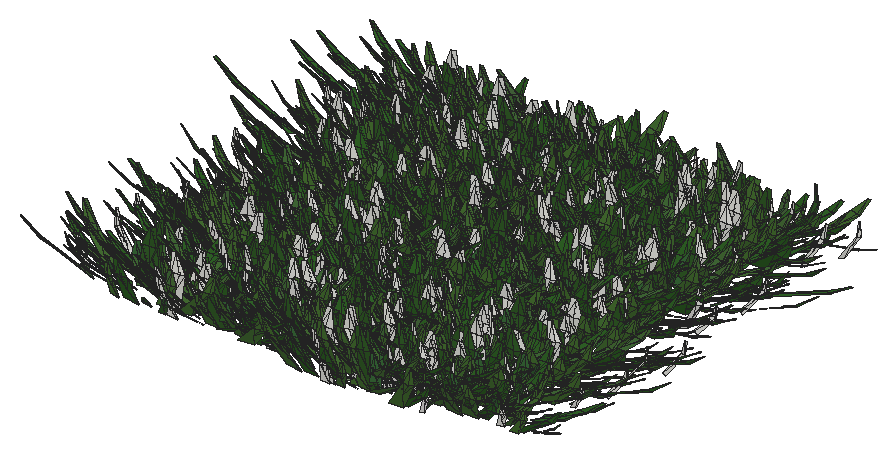
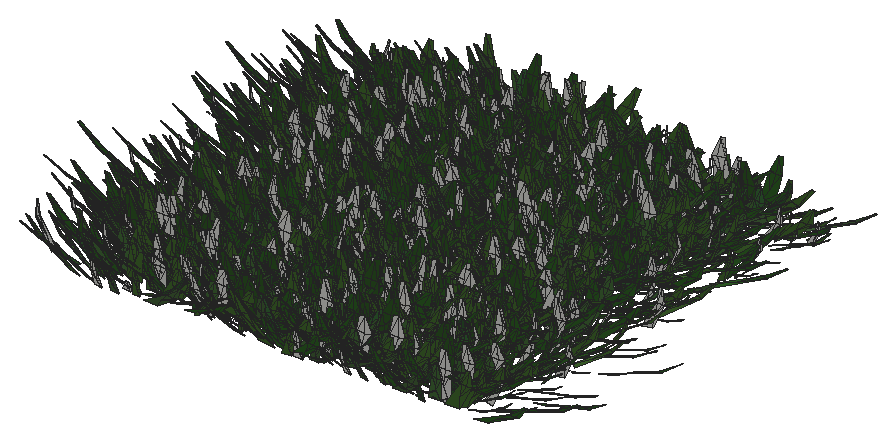
# SketchUp Ruby script. Lengths in inches.
U = 1.inch
M = Sketchup.active_model
def pt(a) = Geom::Point3d.new(a.map { |v| v * U })
def face(e, loops, mat)
  f = e.add_face(loops[0].map { |a| pt(a) })
  loops[1..].each { |l| e.add_face(l.map { |a| pt(a) }).erase! }
  f.material = f.back_material = mat if mat
  f
end
# faces: each face lists its corners as indices into pts; further lists are holes
def faces(e, pts, list, mat = nil) = list.each { |f| face(e, (f[0].is_a?(Array) ? f : [f]).map { |l| l.map { |i| pts[i] } }, mat) }
# xy, xz, yz: faces in a plane at the given z, y or x. An outline is a flat list of corners, or four numbers for a rectangle; further outlines are holes
def ring(l) = l.size == 4 ? [[l[0], l[1]], [l[2], l[1]], [l[2], l[3]], [l[0], l[3]]] : l.each_slice(2).to_a
def flat(e, list, mat, &to3) = list.each { |f| face(e, (f[0].is_a?(Array) ? f : [f]).map { |l| ring(l).map { |u, v| to3.(u, v) } }, mat) }
def xy(e, z, list, mat = nil) = flat(e, list, mat) { |x, y| [x, y, z] }
def xz(e, y, list, mat = nil) = flat(e, list, mat) { |x, z| [x, y, z] }
def yz(e, x, list, mat = nil) = flat(e, list, mat) { |y, z| [x, y, z] }
def lines(e, pts, list) = list.each { |a, b| e.add_line(pt(pts[a]), pt(pts[b])) }
# prism: a flat outline (further loops are holes) pulled along v
def prism(e, loops, v, mat = nil)
  f = face(e, loops, mat); d = Geom::Vector3d.new(v.map { |x| x * U })
  f.pushpull(f.normal.samedirection?(d) ? d.length : -d.length)
end
def box(e, o, s, mat = nil) = prism(e, [[o, [o[0] + s[0], o[1], o[2]], [o[0] + s[0], o[1] + s[1], o[2]], [o[0], o[1] + s[1], o[2]]]], [0, 0, s[2]], mat)
def at(x, y, z, deg = 0) = Geom::Transformation.translation(pt([x, y, z])) * Geom::Transformation.rotation(ORIGIN, Z_AXIS, deg.degrees)
def axes(o, x, y, z) = Geom::Transformation.new([*x, 0, *y, 0, *z, 0, *pt(o).to_a, 1])
def part(name) = M.definitions.add(name)
# library, detail: a bought-in or finely detailed component or shape, given as its bounding box
def library(name, o, s) = part(name).tap { |d| box(d.entities, o, s) }
def detail(e, o, s) = box(e.add_group.entities, o, s)
def put(e, d, t, mat = nil) = e.add_instance(d, t).tap { |i| i.material = mat if mat }
def group(e, t, mat = nil) = e.add_group.tap { |g| g.transformation = t; g.material = mat if mat }.entities
root = M.entities
M.materials.add("Material10").color = [48, 100, 38]
M.materials.add("Material3").color = [68, 110, 58]
M.materials.add("Material4").color = [48, 90, 38]
M.materials.add("Material5").color = [68, 110, 48]
M.materials.add("Material6").color = [48, 90, 48]
M.materials.add("Material7").color = [58, 110, 58]
M.materials.add("Material8").color = [58, 90, 38]
M.materials.add("Material9").color = [68, 100, 58]
c1 = part("grass00")
p = [[-0.6875,0.15,0],[-0.56,0.08,5.52],[-0.04,0.03,2.76],[0.48,-0.02,0],[0.35,-0.02,5.52],[-0.1,-0.14,5.52],
  [-0.12,0.65,8.37],[-0.42,0.65,8.37]]
faces(c1.entities,p,[[0,1,2,3],[3,2,4],[1,5,2],[5,4,2],[1,6,5],[4,5,6],[7,6,1]])
c2 = part("Group16\#1")
put(c2.entities,c1,axes([1.44,-0.61,-0.01],[0.05352,0.12609,0],[-0.10704,0.04543,0.07239],[0.06664,-0.02828,0.11628]),"Material6")
put(c2.entities,c1,axes([0.76,-0.15,-0.01],[0.04676,0.24062,0],[-0.23162,0.04501,0.06642],[0.0652,-0.01267,0.23595]),"Material3")
put(c2.entities,c1,axes([0.79,0.01,-0.01],[-0.00606,0.34651,0],[-0.34381,-0.00602,0.0432],[0.04319,0.00076,0.34386]))
put(c2.entities,c1,axes([1,0.23,-0.01],[-0.07192,0.31144,0],[-0.28722,-0.06632,0.1236],[0.12043,0.02781,0.29478]),"Material5")
put(c2.entities,c1,axes([1.66,0.77,-0.01],[-0.13828,0.29651,0],[-0.21551,-0.1005,0.22471],[0.20365,0.09498,0.23779]),"Material10")
put(c2.entities,c1,axes([0.6875,0.52,-0.01],[-0.18126,0.24051,0],[-0.22746,-0.17142,0.09788],[0.07817,0.05891,0.28481]),"Material5")
put(c2.entities,c1,axes([0.68,0.78,-0.01],[-0.215,0.18688,0],[-0.12385,-0.14248,0.21334],[0.13995,0.16101,0.18878]),"Material3")
put(c2.entities,c1,axes([0.56,1,-0.01],[-0.13756,0.07624,0],[-0.06159,-0.11112,0.0927],[0.04494,0.08108,0.12705]),"Material5")
put(c2.entities,c1,axes([0.2,0.64,-0.01],[-0.23729,0.07254,0],[-0.05711,-0.18681,0.153],[0.04473,0.14632,0.19535]),"Material10")
put(c2.entities,c1,axes([0.0625,0.72,-0.01],[-0.28874,0.02525,0],[-0.02179,-0.24916,0.14647],[0.01276,0.14591,0.25012]),"Material3")
put(c2.entities,c1,axes([-0.08,0.62,-0.01],[-0.34089,-0.04187,0],[0.03255,-0.26504,0.216],[-0.02633,0.21439,0.26703]),"Material10")
put(c2.entities,c1,axes([-0.34,0.98,-0.01],[-0.14314,-0.0493,0],[0.04397,-0.12769,0.06843],[-0.02228,0.0647,0.13505]),"Material10")
put(c2.entities,c1,axes([-0.87,1.45,-0.01],[-0.23488,-0.14114,0],[0.13761,-0.22901,0.06087],[-0.03135,0.05217,0.26717]))
put(c2.entities,c1,axes([-0.72,0.77,-0.01],[-0.14208,-0.13251,0],[0.07209,-0.0773,0.16301],[-0.11118,0.11922,0.1057]),"Material10")
put(c2.entities,c1,axes([-0.62,0.43,-0.01],[-0.14845,-0.21203,0],[0.18654,-0.13061,0.12304],[-0.10079,0.07057,0.22772]),"Material3")
put(c2.entities,c1,axes([-0.68,0.29,-0.01],[-0.13639,-0.32136,0],[0.31723,-0.13464,0.05579],[-0.05136,0.0218,0.34462]),"Material4")
put(c2.entities,c1,axes([-0.64,0.125,-0.01],[-0.0458,-0.23569,0],[0.22124,-0.043,0.08276],[-0.08124,0.01579,0.22538]),"Material7")
put(c2.entities,c1,axes([-1.6,-0.03,-0.01],[0.00576,-0.32897,0],[0.27526,0.00482,0.18018],[-0.18015,-0.00315,0.2753]),"Material5")
put(c2.entities,c1,axes([-1.36,-0.31,-0.01],[0.05718,-0.24765,0],[0.18172,0.04196,0.17267],[-0.16825,-0.03885,0.1865]),"Material10")
put(c2.entities,c1,axes([-1.54,-0.72,-0.01],[0.06537,-0.14017,0],[0.13555,0.06321,0.03939],[-0.0357,-0.01665,0.14956]))
put(c2.entities,c1,axes([-1.19,-0.9,-0.01],[0.09597,-0.12735,0],[0.11214,0.08451,0.07557],[-0.06035,-0.04548,0.14042]),"Material9")
put(c2.entities,c1,axes([-0.47,-0.54,-0.01],[0.11588,-0.10072,0],[0.0618,0.0711,0.12124],[-0.07953,-0.0915,0.0942]))
put(c2.entities,c1,axes([-0.47,-0.84,-0.01],[0.11927,-0.0661,0],[0.06603,0.11913,0.00646],[-0.00313,-0.00565,0.13621]),"Material5")
put(c2.entities,c1,axes([-0.38,-1.24,-0.01],[0.28037,-0.08571,0],[0.0618,0.20215,0.20315],[-0.05939,-0.19428,0.21139]),"Material9")
put(c2.entities,c1,axes([-0.06,-0.66,-0.01],[0.22719,-0.01987,0],[0.01247,0.14255,0.17758],[-0.01547,-0.17691,0.1431]),"Material8")
put(c2.entities,c1,axes([0.11,-0.89,-0.01],[0.14882,0.01828,0],[-0.01058,0.08611,0.12229],[0.01491,-0.12138,0.08676]),"Material6")
put(c2.entities,c1,axes([0.25,-0.72,-0.01],[0.20481,0.07053,0],[-0.06206,0.18022,0.10291],[0.03351,-0.0973,0.1906]),"Material6")
put(c2.entities,c1,axes([0.85,-1.42,-0.01],[0.16481,0.09904,0],[-0.09472,0.15762,0.05616],[0.02893,-0.04814,0.18389]),"Material5")
put(c2.entities,c1,axes([1.01,-1.09,-0.01],[0.21858,0.20385,0],[-0.17495,0.1876,0.15339],[0.10462,-0.11218,0.25652]),"Material10")
put(c2.entities,c1,axes([1.01,-0.71,-0.01],[0.08733,0.12473,0],[-0.06445,0.04512,0.13037],[0.1068,-0.07477,0.07867]),"Material6")
c3 = part("Group15\#1")
put(c3.entities,c2,at(0,0,0))
c4 = part("3darcstudiotree_grass00\#1")
put(c4.entities,c3,at(0,0,0))
put(root,c4,axes([26.17,52.48,7.6],[-3.35209,-0.40812,0],[1.8256,-0.93715,-0.03924],[0.12725,-0.06532,1.93013]))
put(root,c4,axes([26.28,43.875,7.6],[3.10625,-0.85798,0],[3.45102,0.78089,-0.01132],[0.05281,0.01195,1.83032]))
put(root,c4,axes([27.35,67.6875,7.6],[0.47327,-1.08686,0],[4.60722,0.12539,-0.01362],[0.07238,0.00197,1.54899]))
put(root,c4,axes([26.83,70.39,7.6],[-3.67097,0.66942,0],[-2.79157,-0.95678,-0.03459],[-0.12687,-0.04348,1.84283]))
put(root,c4,axes([27.96,75.08,7.6],[-1.67308,-0.99744,0],[3.57228,-0.3745,-0.00949],[0.05914,-0.0062,1.63563]))
put(root,c4,axes([26.8,76.65,7.6],[-2.74123,0.86634,0],[-3.57969,-0.70792,-0.0328],[-0.11955,-0.02364,1.32564]))
put(root,c4,axes([27.89,55.68,7.6],[-4.42043,-0.11266,0],[0.48566,-1.19101,-0.03002],[0.01626,-0.03988,1.59842]))
put(root,c4,axes([27.0625,81.24,7.6],[-1.61796,0.93996,0],[-3.84011,-0.41313,-0.01574],[-0.09207,-0.00991,1.66349]))
put(root,c4,axes([27.55,59.01,7.6],[3.17321,-0.79133,0],[2.66412,0.66769,-0.0036],[0.01703,0.00427,1.5794]))
put(root,c4,axes([26.68,71.74,7.6],[3.39555,0.33213,0],[-1.83469,1.1723,-0.03882],[-0.07009,0.04479,1.55956]))
put(root,c4,axes([27.8,79.22,7.6],[-2.84065,0.70186,0],[-3.36417,-0.85098,-0.01852],[-0.06548,-0.01656,1.50457]))
put(root,c4,axes([27.46,46.76,7.6],[4.32578,-0.20958,0],[0.90693,1.16992,-0.01483],[0.01432,0.01847,1.51152]))
put(root,c4,axes([27.13,61.86,7.6],[3.67456,0.57849,0],[-2.21589,0.8797,-0.03908],[-0.14607,0.05799,1.82303]))
put(root,c4,axes([27.9375,50.86,7.6],[3.12654,0.99148,0],[-3.05993,0.60307,-0.04305],[-0.21095,0.04158,1.51958]))
put(root,c4,axes([30.63,76.96,7.6],[-3.92204,-0.29054,0],[1.17803,-0.99389,-0.05017],[0.08482,-0.07156,1.54202]))
put(root,c4,axes([31.09,70.53,7.6],[-2.30872,-1.02741,0],[3.84342,-0.53979,-0.0488],[0.20495,-0.02878,1.32723]))
put(root,c4,axes([29.8,66.42,7.6],[4.53918,0.22078,0],[-0.91725,1.17863,-0.03864],[-0.04554,0.05852,1.85268]))
put(root,c4,axes([30.03,44.67,7.6],[4.62634,0.00391,0],[-0.01264,0.9349,-0.00416],[-0.00008,0.00596,1.3392]))
put(root,c4,axes([29.99,46.42,7.6],[3.44705,0.83738,0],[-3.43715,0.8843,-0.06236],[-0.26248,0.06753,1.86199]))
put(root,c4,axes([31.96,81.48,7.6],[-2.93,-0.68293,0],[3.05684,-0.81968,-0.04642],[0.17067,-0.04577,1.51042]))
put(root,c4,axes([31.44,64.16,7.6],[1.34292,-0.85261,0],[4.14174,0.40772,-0.0431],[0.19924,0.01961,1.38217]))
put(root,c4,axes([31.49,55.18,7.6],[2.29787,-0.71294,0],[3.86866,0.77932,-0.04335],[0.16802,0.03385,1.54559]))
put(root,c4,axes([32.17,75.38,7.6],[-1.22669,-1.03547,0],[3.63714,-0.2693,-0.01669],[0.12283,-0.00909,1.82011]))
put(root,c4,axes([31.35,52.72,7.6],[-2.98365,0.86497,0],[-3.89047,-0.83874,-0.04683],[-0.20597,-0.0444,1.86493]))
put(root,c4,axes([32.55,73.4,7.6],[-4.10256,-0.1973,0],[0.74416,-0.9671,-0.01319],[0.01782,-0.02316,1.76124]))
put(root,c4,axes([30.78,56.9,7.6],[4.13068,0.36881,0],[-1.71772,1.2024,-0.02984],[-0.04889,0.03422,1.55474]))
put(root,c4,axes([32.57,54.03,7.6],[0.7791,-0.92292,0],[4.72913,0.24951,-0.04294],[0.18667,0.00985,1.34209]))
put(root,c4,axes([33.16,77.8,7.6],[-4.4686,-0.23956,0],[0.88176,-1.02798,-0.03168],[0.03699,-0.04313,1.46389]))
put(root,c4,axes([32.88,58.94,7.6],[1.878,-0.85136,0],[4.01986,0.55421,-0.00061],[0.00361,0.0005,1.94394]))
put(root,c4,axes([33.25,60.34,7.6],[1.24313,-0.92825,0],[4.47227,0.37433,-0.04023],[0.17657,0.01478,1.36415]))
put(root,c4,axes([32.24,63.11,7.6],[-2.14811,0.98739,0],[-4.23231,-0.57547,-0.01158],[-0.04996,-0.00679,1.47884]))
put(root,c4,axes([33.77,67.41,7.6],[-0.51909,-1.27053,0],[4.17352,-0.10657,-0.01024],[0.07103,-0.00181,1.82793]))
put(root,c4,axes([33.17,43.86,7.6],[-2.15627,0.7748,0],[-3.75013,-0.65229,-0.02835],[-0.11927,-0.02075,1.46355]))
put(root,c4,axes([32.47,69.33,7.6],[-0.2443,0.90017,0],[-4.80232,-0.08146,-0.00038],[-0.00184,-0.00003,1.44006]))
put(root,c4,axes([32.82,71.58,7.6],[3.055,0.70222,0],[-2.89109,0.7861,-0.04265],[-0.20546,0.05586,1.90027]))
put(root,c4,axes([33.14,61.48,7.6],[-2.4391,1.11365,0],[-4.52145,-0.61893,-0.00813],[-0.02921,-0.004,1.31962]))
put(root,c4,axes([33.52,50.68,7.6],[-2.85701,0.97241,0],[-3.78392,-0.69484,-0.02364],[-0.12588,-0.02312,1.93862]))
put(root,c4,axes([33.93,49.92,7.6],[3.76686,-0.83119,0],[3.36509,0.95314,-0.00351],[0.01175,0.00333,1.60808]))
put(root,c4,axes([33.96,48.31,7.6],[2.81917,-0.76619,0],[3.32904,0.76557,-0.05921],[0.2958,0.06802,1.91907]))
put(root,c4,axes([33.97,79.74,7.6],[-2.30663,1.06552,0],[-4.23551,-0.57306,-0.04902],[-0.25303,-0.03424,1.76654]))
put(root,c4,axes([36.06,61.82,7.6],[-1.10466,-1.04309,0],[4.11781,-0.27255,-0.00114],[0.00731,-0.00048,1.77079]))
put(root,c4,axes([36.38,52.53,7.6],[-4.80824,-0.47237,0],[1.62347,-1.03284,-0.03326],[0.06769,-0.04306,1.54402]))
put(root,c4,axes([36.37,62.78,7.6],[-4.86512,0.05083,0],[-0.1686,-1.00853,-0.02048],[-0.00677,-0.04048,1.99696]))
put(root,c4,axes([35.83,59.86,7.6],[-3.02468,0.58391,0],[-2.63511,-0.85312,-0.02049],[-0.06609,-0.0214,1.42185]))
put(root,c4,axes([36.38,70.74,7.6],[2.33832,-0.89865,0],[3.29868,0.53645,-0.01966],[0.11007,0.0179,1.64285]))
put(root,c4,axes([37.07,76.47,7.6],[-3.01459,0.57554,0],[-2.90712,-0.95168,-0.0597],[-0.23401,-0.07661,1.93343]))
put(root,c4,axes([36.58,80.09,7.6],[-1.87724,0.90474,0],[-4.04075,-0.52401,-0.04385],[-0.19356,-0.0251,1.41492]))
put(root,c4,axes([37.13,71.88,7.6],[-2.76695,1.05816,0],[-3.42506,-0.55976,-0.05029],[-0.32743,-0.05351,1.98932]))
put(root,c4,axes([37.48,68.93,7.6],[1.10502,-1.02921,0],[4.51643,0.30307,-0.05256],[0.2763,0.01854,1.59089]))
put(root,c4,axes([37.96,75.13,7.6],[-0.89548,-0.9705,0],[4.23678,-0.24433,-0.03351],[0.19208,-0.01108,1.59864]))
put(root,c4,axes([36.48,47.99,7.6],[4.62222,-0.11265,0],[0.48715,1.24932,-0.00515],[0.00288,0.00739,1.80879]))
put(root,c4,axes([38.8,45.89,7.6],[-4.55832,-0.10477,0],[0.39974,-1.08695,-0.01686],[0.00782,-0.02126,1.38194]))
put(root,c4,axes([37.36,57.46,7.6],[-0.72748,0.92095,0],[-4.90606,-0.24221,-0.01512],[-0.08825,-0.00436,1.85999]))
put(root,c4,axes([39.07,51.3125,7.6],[1.03269,-0.98427,0],[4.16593,0.27318,-0.01105],[0.06051,0.00397,1.52421]))
put(root,c4,axes([37.49,44.97,7.6],[1.02056,1.16632,0],[-3.98079,0.21771,-0.00261],[-0.01671,0.00091,1.6704]))
put(root,c4,axes([37.49,67.8,7.6],[2.79724,0.70196,0],[-3.39919,0.84659,-0.03194],[-0.10291,0.02563,1.36388]))
put(root,c4,axes([39.77,55.68,7.6],[-4.31262,-0.5264,0],[2.25127,-1.15275,-0.06565],[0.15274,-0.07821,1.70067]))
put(root,c4,axes([39.99,81.44,7.6],[-1.35682,-1.23326,0],[4.57935,-0.31489,-0.02011],[0.12844,-0.00883,1.9663]))
put(root,c4,axes([38.01,58.25,7.6],[-0.08255,1.17083,0],[-4.86044,-0.02142,-0.00958],[-0.04676,-0.00021,1.48335]))
put(root,c4,axes([38.42,73.11,7.6],[4.4348,0.59016,0],[-2.24354,1.0537,-0.02998],[-0.09351,0.04392,1.98098]))
put(root,c4,axes([38.92,49.8125,7.6],[0.34603,1.04205,0],[-3.81852,0.07925,-0.00998],[-0.05603,0.00116,1.34846]))
put(root,c4,axes([39.82,66.52,7.6],[3.30812,-0.80284,0],[2.65209,0.683,-0.02978],[0.12492,0.03217,1.43312]))
put(root,c4,axes([39.22,64.0625,7.6],[3.9282,0.38594,0],[-1.52945,0.97295,-0.02634],[-0.05842,0.03716,1.58474]))
put(root,c4,axes([39.91,53.36,7.6],[3.43387,-0.66059,0],[2.3393,0.76,-0.03629],[0.13053,0.04241,1.41389]))
put(root,c4,axes([40.05,78.42,7.6],[3.76187,0.14522,0],[-0.63051,1.02078,-0.03647],[-0.03383,0.05478,1.56991]))
put(root,c4,axes([41.96,65.59,7.6],[-4.18758,-0.22232,0],[0.96219,-1.13271,-0.02543],[0.02933,-0.03453,1.60712]))
put(root,c4,axes([42.84,61.76,7.6],[-1.50965,-1.02726,0],[3.51869,-0.32319,-0.02344],[0.12593,-0.01157,1.34096]))
put(root,c4,axes([42.66,82.25,7.6],[-4.14711,0.13047,0],[-0.48074,-0.95501,-0.01354],[-0.00996,-0.01978,1.41676]))
put(root,c4,axes([42.59,49.45,7.6],[-3.93065,0.22936,0],[-0.83099,-0.89006,-0.0198],[-0.02909,-0.03116,1.47686]))
put(root,c4,axes([42.41,62.96,7.6],[1.12797,-1.08226,0],[3.79109,0.24695,-0.04641],[0.27021,0.0176,1.47323]))
put(root,c4,axes([43.23,59.81,7.6],[0.07706,-1.18991,0],[5.14858,0.02084,-0.02796],[0.13847,0.00056,1.59394]))
put(root,c4,axes([43.34,58.04,7.6],[-4.65628,0.436,0],[-1.28176,-0.85553,-0.01358],[-0.03081,-0.02057,1.47772]))
put(root,c4,axes([43.74,56.96,7.6],[-4.55351,-0.01078,0],[0.04878,-1.28737,-0.04475],[0.00189,-0.04985,1.43393]))
put(root,c4,axes([43.03,67.88,7.6],[3.27668,-0.61327,0],[2.78187,0.92896,-0.01707],[0.06911,0.02308,1.96039]))
put(root,c4,axes([43.96,55.76,7.6],[-4.03083,-0.21133,0],[0.96222,-1.14709,-0.00999],[0.00968,-0.01153,1.38276]))
put(root,c4,axes([42.52,73.625,7.6],[4.2465,-0.26624,0],[0.87998,0.87721,-0.03452],[0.06922,0.06901,1.86367]))
put(root,c4,axes([43.5625,65.09,7.6],[-2.58663,0.93393,0],[-3.19563,-0.55317,-0.03104],[-0.18757,-0.03247,1.78553]))
put(root,c4,axes([44.08,47.88,7.6],[3.25384,-0.82472,0],[2.88656,0.71179,-0.00165],[0.00841,0.00207,1.81884]))
put(root,c4,axes([43.29,71.82,7.6],[4.50216,0.32859,0],[-1.15691,0.9907,-0.03197],[-0.04777,0.04091,1.37583]))
put(root,c4,axes([45.35,79.77,7.6],[-3.56236,-0.42367,0],[2.09245,-1.09962,-0.03826],[0.09877,-0.05191,1.82966]))
put(root,c4,axes([45.22,44.79,7.6],[-1.82775,-1.1638,0],[4.23116,-0.41531,-0.05278],[0.32118,-0.03153,1.85719]))
put(root,c4,axes([45.34,45.84,7.6],[-4.77315,-0.10069,0],[0.4015,-1.18962,-0.02802],[0.01422,-0.04212,1.8014]))
put(root,c4,axes([43.91,53.65,7.6],[4.00974,0.00197,0],[-0.00725,0.92038,-0.0306],[-0.0005,0.06325,1.9022]))
put(root,c4,axes([45.46,52.69,7.6],[-3.72919,-0.05138,0],[0.24763,-1.12327,-0.00601],[0.00211,-0.00957,1.79325]))
put(root,c4,axes([45.55,76.17,7.6],[1.19738,-1.09661,0],[4.52965,0.30912,-0.00598],[0.02664,0.00182,1.35627]))
put(root,c4,axes([44.76,75.65,7.6],[3.65568,-0.70914,0],[2.22099,0.71559,-0.00126],[0.00457,0.00147,1.3431]))
put(root,c4,axes([45.16,80.75,7.6],[2.61731,-0.86986,0],[3.89148,0.73181,-0.05537],[0.21942,0.04126,1.50911]))
put(root,c4,axes([44.58,77.9375,7.6],[3.93859,-0.14638,0],[0.69101,1.16209,-0.00967],[0.00686,0.01153,1.41667]))
put(root,c4,axes([44.36,43.44,7.6],[1.45046,1.05694,0],[-4.51111,0.38692,-0.02597],[-0.16209,0.0139,1.96681]))
put(root,c4,axes([44.36,51.22,7.6],[3.4597,0.79761,0],[-3.28778,0.89131,-0.03053],[-0.13377,0.03626,1.95907]))
put(root,c4,axes([45.58,70.75,7.6],[-2.65201,0.65355,0],[-3.42376,-0.86832,-0.05994],[-0.20928,-0.05308,1.51606]))
put(root,c4,axes([44.67,69.22,7.6],[2.03961,1.07438,0],[-3.7474,0.44463,-0.01135],[-0.07143,0.00848,1.80626]))
put(root,c4,axes([48.18,69.59,7.6],[-4.36276,-0.41418,0],[1.61781,-1.06507,-0.04397],[0.10568,-0.06958,1.92843]))
put(root,c4,axes([47.6875,46.17,7.6],[4.18598,-0.49036,0],[1.98476,1.05894,-0.00986],[0.01957,0.01044,1.36783]))
put(root,c4,axes([48.1875,79.875,7.6],[2.56056,-0.98432,0],[3.11203,0.50597,-0.04791],[0.30541,0.04966,1.76421]))
put(root,c4,axes([48.4375,43.4,7.6],[-2.25026,0.83212,0],[-3.28634,-0.55544,-0.04556],[-0.29795,-0.05036,1.95702]))
put(root,c4,axes([47.9375,70.16,7.6],[4.24107,-0.51199,0],[1.69937,0.8798,-0.04306],[0.14953,0.07741,1.95064]))
put(root,c4,axes([48.74,58.24,7.6],[-3.84253,0.80536,0],[-2.94777,-0.87903,-0.04843],[-0.1539,-0.04589,1.41858]))
put(root,c4,axes([48.07,54.37,7.6],[3.94053,-0.29196,0],[1.05758,0.89211,-0.03127],[0.05685,0.04795,1.48816]))
put(root,c4,axes([48.08,52.59,7.6],[-1.53168,1.15293,0],[-4.14234,-0.34395,-0.00679],[-0.03089,-0.00256,1.30662]))
put(root,c4,axes([48.95,61.6,7.6],[2.91217,-0.96079,0],[3.36935,0.63829,-0.04967],[0.26034,0.04932,1.73743]))
put(root,c4,axes([48.26,73.77,7.6],[3.5038,0.25818,0],[-1.36394,1.15688,-0.04213],[-0.05636,0.0478,1.42653]))
put(root,c4,axes([48.28,49.08,7.6],[3.5404,0.59381,0],[-2.40006,0.89434,-0.0468],[-0.15546,0.05793,1.60535]))
put(root,c4,axes([49.06,72.07,7.6],[0.13139,0.97083,0],[-4.91867,0.04161,-0.06181],[-0.35555,0.00301,1.77032]))
put(root,c4,axes([50.17,67.81,7.6],[0.40983,-1.2299,0],[4.04007,0.08414,-0.04948],[0.34314,0.00715,1.76318]))
put(root,c4,axes([49.5,66.11,7.6],[-1.3481,0.99436,0],[-4.38162,-0.37127,-0.05878],[-0.26746,-0.02266,1.38915]))
put(root,c4,axes([50.9,64.74,7.6],[-4.22259,-0.42472,0],[1.51539,-0.94162,-0.02256],[0.05153,-0.03202,1.55256]))
put(root,c4,axes([49.27,62.65,7.6],[5.02289,-0.20794,0],[0.8428,1.27239,-0.06031],[0.06068,0.09161,1.9859]))
put(root,c4,axes([49,76.65,7.6],[3.33218,0.8255,0],[-3.60999,0.91074,-0.05903],[-0.23844,0.06015,1.83956]))
put(root,c4,axes([48.96,56.43,7.6],[2.8431,0.99871,0],[-3.14486,0.55954,-0.01154],[-0.05137,0.00914,1.31865]))
put(root,c4,axes([50.63,47.89,7.6],[0.55232,-1.11163,0],[4.16686,0.1294,-0.05019],[0.29048,0.00902,1.53052]))
put(root,c4,axes([50.01,80.9,7.6],[-1.89808,0.89436,0],[-4.05381,-0.53771,-0.05129],[-0.21186,-0.0281,1.34106]))
put(root,c4,axes([49.86,60.36,7.6],[3.55839,0.29687,0],[-1.56966,1.17589,-0.04175],[-0.06486,0.04859,1.52086]))
put(root,c4,axes([51.91,78.11,7.6],[-3.54234,-0.75482,0],[2.45019,-0.71866,-0.02002],[0.0717,-0.02103,1.30322]))
put(root,c4,axes([50.26,50.54,7.6],[4.48344,-0.16058,0],[0.51704,0.90226,-0.032],[0.03977,0.0694,1.99674]))
put(root,c4,axes([50.74,45.05,7.6],[1.95173,0.87312,0],[-3.39618,0.47448,-0.02391],[-0.12805,0.01789,1.49173]))
put(root,c4,axes([50.75,55.31,7.6],[0.71334,1.19036,0],[-4.87402,0.18255,-0.01905],[-0.09604,0.0036,1.57029]))
put(root,c4,axes([51.59,75.2,7.6],[4.42918,0.20065,0],[-0.79517,1.09706,-0.0513],[-0.05083,0.07012,1.54883]))
put(root,c4,axes([54.34,66.32,7.6],[-3.33998,-0.7783,0],[3.18573,-0.85444,-0.00052],[0.00217,-0.00058,1.79691]))
put(root,c4,axes([54.34,79.92,7.6],[0.94379,-0.92824,0],[3.72731,0.23686,-0.00558],[0.03773,0.0024,1.6757]))
put(root,c4,axes([54.26,74.71,7.6],[2.03979,-0.89321,0],[3.8754,0.55313,-0.00497],[0.021,0.003,1.35772]))
put(root,c4,axes([54.58,77.18,7.6],[2.39407,-0.96093,0],[3.77709,0.58814,-0.04551],[0.23245,0.0362,1.67334]))
put(root,c4,axes([54.37,68.1,7.6],[2.46437,0.8072,0],[-2.94216,0.5614,-0.04536],[-0.29999,0.05724,1.92466]))
put(root,c4,axes([54.7,81.47,7.6],[-1.30402,1.0923,0],[-3.59141,-0.26797,-0.00408],[-0.02313,-0.00173,1.38631]))
put(root,c4,axes([55.95,69.47,7.6],[-0.13657,-1.25054,0],[5.17112,-0.0353,-0.06757],[0.36478,-0.00249,1.74608]))
put(root,c4,axes([56.15,64.68,7.6],[0.26147,-1.07741,0],[4.77538,0.07243,-0.04584],[0.20115,0.00305,1.3146]))
put(root,c4,axes([56.4375,52.6,7.6],[-0.00527,-1.07979,0],[5.08619,-0.00155,-0.02113],[0.09419,-0.00003,1.41674]))
put(root,c4,axes([54.98,47.6875,7.6],[3.80252,-0.21307,0],[0.8211,0.91584,-0.01015],[0.01463,0.01631,1.54623]))
put(root,c4,axes([54.94,49.08,7.6],[-1.38358,0.95904,0],[-3.87916,-0.34977,-0.00809],[-0.05318,-0.0048,1.80065]))
put(root,c4,axes([56.67,82.68,7.6],[-2.64683,-0.75591,0],[3.71627,-0.81329,-0.03006],[0.12697,-0.02779,1.73276]))
put(root,c4,axes([55.65,53.71,7.6],[3.22127,-0.6295,0],[2.94777,0.94277,-0.00613],[0.02206,0.00705,1.74641]))
put(root,c4,axes([54.84,62.48,7.6],[0.12956,0.95583,0],[-3.83664,0.0325,-0.00216],[-0.01582,0.00013,1.758]))
put(root,c4,axes([56.33,78.41,7.6],[0.29566,-0.96452,0],[4.47879,0.08581,-0.05496],[0.37486,0.00718,1.9204]))
put(root,c4,axes([56.65,55.99,7.6],[-0.81018,-1.00031,0],[4.10104,-0.2076,-0.04711],[0.26622,-0.01348,1.50792]))
put(root,c4,axes([55.74,70.89,7.6],[3.64126,-0.56822,0],[2.32111,0.92964,-0.03499],[0.12777,0.05117,1.88939]))
put(root,c4,axes([56.09,59.7,7.6],[2.71786,-0.72349,0],[3.02088,0.70927,-0.02466],[0.11069,0.02599,1.59511]))
put(root,c4,axes([55.92,50.92,7.6],[-3.07818,0.70756,0],[-3.19663,-0.86917,-0.0061],[-0.02564,-0.00697,1.83281]))
put(root,c4,axes([55.84,46.01,7.6],[-1.05333,1.02923,0],[-4.06109,-0.25976,-0.04208],[-0.23965,-0.01533,1.54007]))
put(root,c4,axes([57.45,58.43,7.6],[-0.35317,-0.93176,0],[5.0183,-0.11888,-0.03587],[0.18182,-0.00431,1.60406]))
put(root,c4,axes([55.92,73.17,7.6],[4.77949,0.09804,0],[-0.30213,0.92053,-0.01884],[-0.00915,0.02789,1.37151]))
put(root,c4,axes([55.8,72.48,7.6],[3.18507,0.78996,0],[-2.86494,0.72195,-0.02475],[-0.11175,0.02816,1.62992]))
put(root,c4,axes([56.06,45.33,7.6],[4.28562,0.46278,0],[-1.51887,0.87911,-0.02193],[-0.0534,0.03091,1.47013]))
